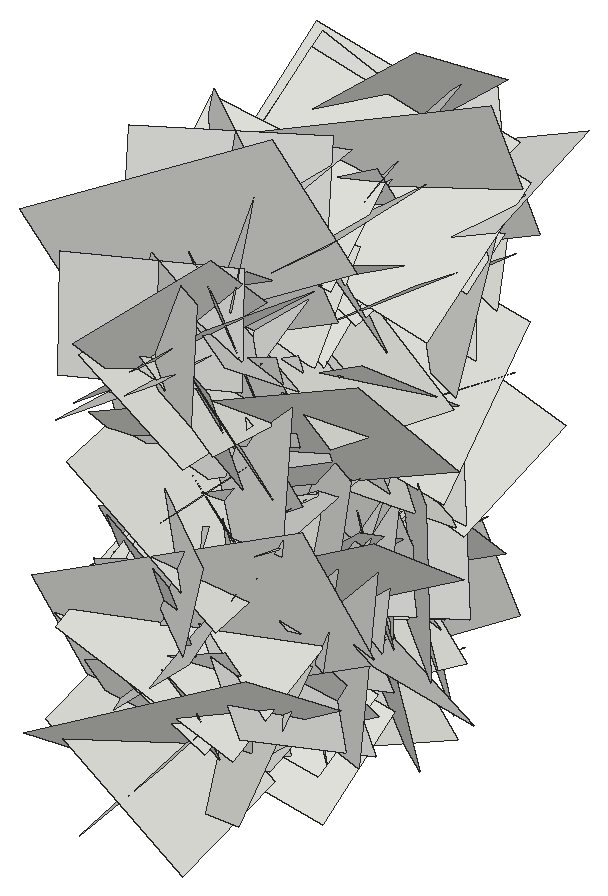
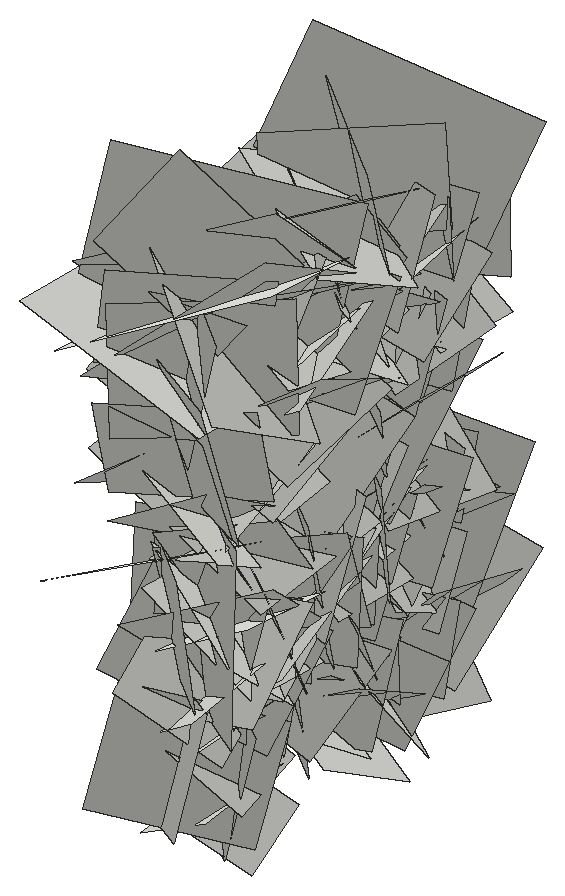
# SketchUp Ruby script. Lengths in inches.
U = 1.inch
M = Sketchup.active_model
def pt(a) = Geom::Point3d.new(a.map { |v| v * U })
def face(e, loops, mat)
  f = e.add_face(loops[0].map { |a| pt(a) })
  loops[1..].each { |l| e.add_face(l.map { |a| pt(a) }).erase! }
  f.material = f.back_material = mat if mat
  f
end
# faces: each face lists its corners as indices into pts; further lists are holes
def faces(e, pts, list, mat = nil) = list.each { |f| face(e, (f[0].is_a?(Array) ? f : [f]).map { |l| l.map { |i| pts[i] } }, mat) }
# xy, xz, yz: faces in a plane at the given z, y or x. An outline is a flat list of corners, or four numbers for a rectangle; further outlines are holes
def ring(l) = l.size == 4 ? [[l[0], l[1]], [l[2], l[1]], [l[2], l[3]], [l[0], l[3]]] : l.each_slice(2).to_a
def flat(e, list, mat, &to3) = list.each { |f| face(e, (f[0].is_a?(Array) ? f : [f]).map { |l| ring(l).map { |u, v| to3.(u, v) } }, mat) }
def xy(e, z, list, mat = nil) = flat(e, list, mat) { |x, y| [x, y, z] }
def xz(e, y, list, mat = nil) = flat(e, list, mat) { |x, z| [x, y, z] }
def yz(e, x, list, mat = nil) = flat(e, list, mat) { |y, z| [x, y, z] }
def lines(e, pts, list) = list.each { |a, b| e.add_line(pt(pts[a]), pt(pts[b])) }
# prism: a flat outline (further loops are holes) pulled along v
def prism(e, loops, v, mat = nil)
  f = face(e, loops, mat); d = Geom::Vector3d.new(v.map { |x| x * U })
  f.pushpull(f.normal.samedirection?(d) ? d.length : -d.length)
end
def box(e, o, s, mat = nil) = prism(e, [[o, [o[0] + s[0], o[1], o[2]], [o[0] + s[0], o[1] + s[1], o[2]], [o[0], o[1] + s[1], o[2]]]], [0, 0, s[2]], mat)
def at(x, y, z, deg = 0) = Geom::Transformation.translation(pt([x, y, z])) * Geom::Transformation.rotation(ORIGIN, Z_AXIS, deg.degrees)
def axes(o, x, y, z) = Geom::Transformation.new([*x, 0, *y, 0, *z, 0, *pt(o).to_a, 1])
def part(name) = M.definitions.add(name)
# library, detail: a bought-in or finely detailed component or shape, given as its bounding box
def library(name, o, s) = part(name).tap { |d| box(d.entities, o, s) }
def detail(e, o, s) = box(e.add_group.entities, o, s)
def put(e, d, t, mat = nil) = e.add_instance(d, t).tap { |i| i.material = mat if mat }
def group(e, t, mat = nil) = e.add_group.tap { |g| g.transformation = t; g.material = mat if mat }.entities
root = M.entities
c1 = part("Component\#6")
p = [[0.01,0,0],[0,3.24,4.54],[4.32,3.24,4.54],[4.33,0,0]]
faces(c1.entities,p,[[0,1,2,3]])
put(root,c1,axes([34.14,153.52,29.46],[-0.08102,0.00764,-0.81457],[-0.10707,-0.81193,0.00187],[0.85682,-0.10074,-0.07679]))
put(root,c1,axes([34.14,158.01,30.39],[0.08038,-0.60995,0.00551],[-0.02253,0.00291,0.6143],[0.64618,0.07598,0.02073]))
put(root,c1,axes([34.14,151.89,27.92],[0.07457,-0.37507,-0.49968],[-0.035,-0.50437,0.37394],[0.66135,0.0156,0.07613]))
put(root,c1,axes([38.11,158.65,23.12],[0.03,-0.65446,0.65644],[-0.11713,0.64968,0.65248],[-0.97555,-0.09812,-0.05816]))
put(root,c1,axes([34.14,150.81,32.67],[-0.03105,-0.70657,0.01303],[0.00041,0.01303,0.70717],[0.74909,-0.02929,0.00015]))
put(root,c1,axes([38.11,155.99,38.05],[-0.0315,0.52335,-0.79271],[0.01447,-0.79278,-0.52391],[-1.00678,-0.02777,0.01727]))
put(root,c1,axes([34.14,155.3,36.05],[-0.02231,-0.46484,-0.62566],[-0.10069,-0.6197,0.4636],[0.82005,-0.08874,0.0399]))
put(root,c1,axes([38.11,160.9375,37.33],[-0.13153,0.12633,-0.90974],[0.10231,-0.91113,-0.13969],[-0.96819,-0.11344,0.10882]))
put(root,c1,axes([38.11,153.79,24.7],[0.00565,-0.43188,0.90191],[0.04751,0.90112,0.43124],[-1.05892,0.03812,0.02416]))
put(root,c1,axes([38.11,152.27,30.34],[-0.04267,0.47891,-0.74389],[-0.05776,-0.74459,-0.47642],[-0.93603,0.02411,0.06331]))
put(root,c1,axes([38.11,150.92,33.45],[0.01124,-0.40239,0.85237],[-0.02564,0.85203,0.40253],[-0.99881,-0.0264,-0.00074]))
put(root,c1,axes([34.14,153.82,25.23],[0.04726,-0.11023,0.59197],[0.093,0.58845,0.10297],[0.63147,-0.07841,-0.05947]))
put(root,c1,axes([34.14,149.71,29.1],[0.04042,0.22115,-0.567],[0.10046,-0.56334,-0.21335],[0.63725,0.07479,0.0696]))
put(root,c1,axes([38.11,154.45,36.57],[-0.07713,0.81709,0.22722],[-0.03645,0.22503,-0.82021],[-0.89825,-0.07929,0.01378]))
put(root,c1,axes([34.14,158.75,26.14],[0.12859,0.59437,-0.23179],[-0.06253,-0.22448,-0.60651],[0.67335,-0.13435,-0.01206]))
put(root,c1,axes([38.11,156.72,22.08],[0.00521,-0.94479,0.50901],[0.17637,0.50353,0.93301],[-1.12382,0.07464,0.14878]))
put(root,c1,axes([34.14,156.34,37.48],[-0.20366,-0.78098,-0.33642],[0.07649,-0.35863,0.79133],[0.89812,-0.14656,-0.14368]))
put(root,c1,axes([38.11,150.56,37.37],[-0.01495,0.72639,-0.4873],[-0.06872,-0.48689,-0.7239],[-0.92463,0.02444,0.06168]))
put(root,c1,axes([34.14,156.49,28.09],[0.01227,0.36562,0.53928],[0.0952,0.53332,-0.36351],[0.68404,-0.08079,0.04092]))
put(root,c1,axes([38.11,150.4,30.92],[-0.04252,-0.27759,0.76161],[-0.13298,0.75548,0.26875],[-0.84891,-0.10444,-0.08025]))
put(root,c1,axes([38.11,152.31,24.83],[-0.14132,0.38772,0.61473],[-0.11706,0.60692,-0.40674],[-0.76145,-0.16526,-0.05156]))
put(root,c1,axes([34.14,150.69,21.46],[-0.08617,-0.06424,0.73191],[0.1147,0.7273,0.07585],[0.77031,-0.11548,0.07058]))
put(root,c1,axes([34.14,149.63,26.39],[-0.05575,0.3601,-0.58557],[0.15834,-0.56726,-0.36226],[0.71127,0.15451,0.03475]))
put(root,c1,axes([34.14,153.92,21.15],[-0.0271,-0.2919,0.8704],[-0.20523,0.85287,0.28034],[0.95124,0.17569,0.08528]))
put(root,c1,axes([34.14,159.1875,20.3125],[-0.01409,-0.35632,0.80543],[-0.16766,0.79339,0.34838],[0.91839,0.13938,0.07596]))
put(root,c1,axes([38.11,157.73,31.39],[0.13129,-0.92283,0.37392],[-0.04334,0.37177,0.93107],[-1.05456,-0.13017,0.00829]))
put(root,c1,axes([34.14,147.16,24.1],[-0.03025,0.92414,0.23442],[-0.23339,0.2218,-0.90118],[0.98329,0.08108,-0.20669]))
put(root,c1,axes([34.14,159.76,21.63],[0.09665,-0.666,0.12875],[-0.03078,0.12595,0.67212],[0.71837,0.095,0.01147]))
put(root,c1,axes([38.11,154.61,36.92],[0.07328,1.03426,0.55463],[0.26621,0.52968,-1.01904],[-1.21518,0.17841,-0.1898]))
put(root,c1,axes([34.14,160.84,30.26],[0.09118,-0.56201,-0.30691],[0.0596,-0.30185,0.56849],[0.67615,0.1024,-0.00872]))
put(root,c1,axes([34.14,156.05,22.34],[0.04217,-0.56806,-0.37659],[0.07293,-0.37196,0.56834],[0.71876,0.07107,-0.03557]))
put(root,c1,axes([38.11,158.82,28.52],[0.0834,-0.34729,-0.88838],[-0.00654,-0.89156,0.34799],[-1.01106,-0.02288,-0.07553]))
put(root,c1,axes([38.11,151.53,22],[0.08087,0.78957,0.40941],[-0.10212,0.41583,-0.78401],[-0.93722,0.02282,0.12075]))
put(root,c1,axes([38.11,152.86,25.21],[-0.07237,-0.84668,-0.40971],[0.16913,-0.41526,0.83156],[-0.98259,-0.00911,0.17331]))
put(root,c1,axes([38.11,150.44,37.52],[0.01758,-0.03984,-0.83316],[-0.08726,-0.82933,0.03802],[-0.87984,0.08145,-0.02042]))
put(root,c1,axes([38.11,161.57,34.4],[0.05292,-0.24359,-0.78611],[-0.1523,-0.77804,0.23197],[-0.85897,0.12294,-0.08956]))
put(root,c1,axes([34.14,154.14,39.875],[-0.07687,-0.17009,-0.90128],[-0.07958,-0.89996,0.17589],[0.96896,-0.0874,-0.05706]))
put(root,c1,axes([34.14,159.35,19.53],[0.12506,-0.65018,0.20227],[-0.00025,0.20525,0.65988],[0.72178,0.11273,-0.03482]))
put(root,c1,axes([38.11,155.63,34.51],[0.04715,-0.7148,-0.47013],[-0.06325,-0.47221,0.71232],[-0.90467,-0.00424,-0.0743]))
put(root,c1,axes([38.11,151.43,29.49],[0.01376,0.93036,0.01045],[0.09599,0.00914,-0.92605],[-0.98156,0.01394,-0.09041]))
put(root,c1,axes([38.11,156.02,27.27],[-0.01737,0.78195,0.05447],[-0.0729,0.05284,-0.77921],[-0.82768,-0.02106,0.06749]))
put(root,c1,axes([34.14,152.23,36.27],[0.17612,0.33723,0.58016],[-0.03508,0.60107,-0.33991],[0.71045,-0.05392,-0.16061]))
put(root,c1,axes([34.14,152.86,32.22],[-0.07765,-0.95123,0.12327],[-0.10469,0.13045,0.94796],[1.01133,-0.05954,0.1076]))
put(root,c1,axes([38.11,160.42,26.72],[0.04031,-0.6417,-0.5437],[-0.04231,-0.54502,0.64047],[-0.89052,-0.00315,-0.05504]))
put(root,c1,axes([34.14,153.18,27.99],[-0.08911,-1.01671,-0.11332],[-0.1646,-0.0997,1.00972],[1.07181,-0.09984,0.14565]))
put(root,c1,axes([38.11,153.18,27.99],[0.08911,-1.01671,-0.11332],[0.1646,-0.0997,1.00972],[-1.07181,-0.09984,0.14565]))
put(root,c1,axes([34.14,160.42,26.72],[-0.04031,-0.6417,-0.5437],[0.04231,-0.54502,0.64047],[0.89052,-0.00315,-0.05504]))
put(root,c1,axes([38.11,152.86,32.22],[0.07765,-0.95123,0.12327],[0.10469,0.13045,0.94796],[-1.01133,-0.05954,0.1076]))
put(root,c1,axes([38.11,152.23,36.27],[-0.17612,0.33723,0.58016],[0.03508,0.60107,-0.33991],[-0.71045,-0.05392,-0.16061]))
put(root,c1,axes([34.14,156.02,27.27],[0.01737,0.78195,0.05447],[0.0729,0.05284,-0.77921],[0.82768,-0.02106,0.06749]))
put(root,c1,axes([34.14,151.43,29.49],[-0.01376,0.93036,0.01045],[-0.09599,0.00914,-0.92605],[0.98156,0.01394,-0.09041]))
put(root,c1,axes([34.14,155.63,34.51],[-0.04715,-0.7148,-0.47013],[0.06325,-0.47221,0.71232],[0.90467,-0.00424,-0.0743]))
put(root,c1,axes([38.11,159.35,19.53],[-0.12506,-0.65018,0.20227],[0.00025,0.20525,0.65988],[-0.72178,0.11273,-0.03482]))
put(root,c1,axes([38.11,154.14,39.875],[0.07687,-0.17009,-0.90128],[0.07958,-0.89996,0.17589],[-0.96896,-0.0874,-0.05706]))
put(root,c1,axes([34.14,161.57,34.4],[-0.05292,-0.24359,-0.78611],[0.1523,-0.77804,0.23197],[0.85897,0.12294,-0.08956]))
put(root,c1,axes([34.14,150.44,37.52],[-0.01758,-0.03984,-0.83316],[0.08726,-0.82933,0.03802],[0.87984,0.08145,-0.02042]))
put(root,c1,axes([34.14,152.86,25.21],[0.07237,-0.84668,-0.40971],[-0.16913,-0.41526,0.83156],[0.98259,-0.00911,0.17331]))
put(root,c1,axes([34.14,151.53,22],[-0.08087,0.78957,0.40941],[0.10212,0.41583,-0.78401],[0.93722,0.02282,0.12075]))
put(root,c1,axes([34.14,158.82,28.52],[-0.0834,-0.34729,-0.88838],[0.00654,-0.89156,0.34799],[1.01106,-0.02288,-0.07553]))
put(root,c1,axes([38.11,156.05,22.34],[-0.04217,-0.56806,-0.37659],[-0.07293,-0.37196,0.56834],[-0.71876,0.07107,-0.03557]))
put(root,c1,axes([38.11,160.84,30.26],[-0.09118,-0.56201,-0.30691],[-0.0596,-0.30185,0.56849],[-0.67615,0.1024,-0.00872]))
put(root,c1,axes([34.14,154.61,36.92],[-0.07328,1.03426,0.55463],[-0.26621,0.52968,-1.01904],[1.21518,0.17841,-0.1898]))
put(root,c1,axes([38.11,159.76,21.63],[-0.09665,-0.666,0.12875],[0.03078,0.12595,0.67212],[-0.71837,0.095,0.01147]))
put(root,c1,axes([38.11,147.16,24.1],[0.03025,0.92414,0.23442],[0.23339,0.2218,-0.90118],[-0.98329,0.08108,-0.20669]))
put(root,c1,axes([34.14,157.73,31.39],[-0.13129,-0.92283,0.37392],[0.04334,0.37177,0.93107],[1.05456,-0.13017,0.00829]))
put(root,c1,axes([38.11,159.1875,20.3125],[0.01409,-0.35632,0.80543],[0.16766,0.79339,0.34838],[-0.91839,0.13938,0.07596]))
put(root,c1,axes([38.11,153.92,21.15],[0.0271,-0.2919,0.8704],[0.20523,0.85287,0.28034],[-0.95124,0.17569,0.08528]))
put(root,c1,axes([38.11,149.63,26.39],[0.05575,0.3601,-0.58557],[-0.15834,-0.56726,-0.36226],[-0.71127,0.15451,0.03475]))
put(root,c1,axes([38.11,150.69,21.46],[0.08617,-0.06424,0.73191],[-0.1147,0.7273,0.07585],[-0.77031,-0.11548,0.07058]))
put(root,c1,axes([34.14,152.31,24.83],[0.14132,0.38772,0.61473],[0.11706,0.60692,-0.40674],[0.76145,-0.16526,-0.05156]))
put(root,c1,axes([34.14,150.4,30.92],[0.04252,-0.27759,0.76161],[0.13298,0.75548,0.26875],[0.84891,-0.10444,-0.08025]))
put(root,c1,axes([38.11,156.49,28.09],[-0.01227,0.36562,0.53928],[-0.0952,0.53332,-0.36351],[-0.68404,-0.08079,0.04092]))
put(root,c1,axes([34.14,150.56,37.37],[0.01495,0.72639,-0.4873],[0.06872,-0.48689,-0.7239],[0.92463,0.02444,0.06168]))
put(root,c1,axes([38.11,156.34,37.48],[0.20366,-0.78098,-0.33642],[-0.07649,-0.35863,0.79133],[-0.89812,-0.14656,-0.14368]))
put(root,c1,axes([34.14,156.72,22.08],[-0.00521,-0.94479,0.50901],[-0.17637,0.50353,0.93301],[1.12382,0.07464,0.14878]))
put(root,c1,axes([38.11,158.75,26.14],[-0.12859,0.59437,-0.23179],[0.06253,-0.22448,-0.60651],[-0.67335,-0.13435,-0.01206]))
put(root,c1,axes([34.14,154.45,36.57],[0.07713,0.81709,0.22722],[0.03645,0.22503,-0.82021],[0.89825,-0.07929,0.01378]))
put(root,c1,axes([38.11,149.71,29.1],[-0.04042,0.22115,-0.567],[-0.10046,-0.56334,-0.21335],[-0.63725,0.07479,0.0696]))
put(root,c1,axes([38.11,153.82,25.23],[-0.04726,-0.11023,0.59197],[-0.093,0.58845,0.10297],[-0.63147,-0.07841,-0.05947]))
put(root,c1,axes([34.14,150.92,33.45],[-0.01124,-0.40239,0.85237],[0.02564,0.85203,0.40253],[0.99881,-0.0264,-0.00074]))
put(root,c1,axes([34.14,152.27,30.34],[0.04267,0.47891,-0.74389],[0.05776,-0.74459,-0.47642],[0.93603,0.02411,0.06331]))
put(root,c1,axes([34.14,153.79,24.7],[-0.00565,-0.43188,0.90191],[-0.04751,0.90112,0.43124],[1.05892,0.03812,0.02416]))
put(root,c1,axes([34.14,160.9375,37.33],[0.13153,0.12633,-0.90974],[-0.10231,-0.91113,-0.13969],[0.96819,-0.11344,0.10882]))
put(root,c1,axes([38.11,155.3,36.05],[0.02231,-0.46484,-0.62566],[0.10069,-0.6197,0.4636],[-0.82005,-0.08874,0.0399]))
put(root,c1,axes([34.14,155.99,38.05],[0.0315,0.52335,-0.79271],[-0.01447,-0.79278,-0.52391],[1.00678,-0.02777,0.01727]))
put(root,c1,axes([38.11,150.81,32.67],[0.03105,-0.70657,0.01303],[-0.00041,0.01303,0.70717],[-0.74909,-0.02929,0.00015]))
put(root,c1,axes([34.14,158.65,23.12],[-0.03,-0.65446,0.65644],[0.11713,0.64968,0.65248],[0.97555,-0.09812,-0.05816]))
put(root,c1,axes([38.11,151.89,27.92],[-0.07457,-0.37507,-0.49968],[0.035,-0.50437,0.37394],[-0.66135,0.0156,0.07613]))
put(root,c1,axes([38.11,158.01,30.39],[-0.08038,-0.60995,0.00551],[0.02253,0.00291,0.6143],[-0.64618,0.07598,0.02073]))
put(root,c1,axes([38.11,153.52,29.46],[0.08102,0.00764,-0.81457],[0.10707,-0.81193,0.00187],[-0.85682,-0.10074,-0.07679]))
put(root,c1,axes([34.14,152.65,32.7],[-0.31384,1.21799,0.62272],[-0.13011,0.61092,-1.25326],[1.44417,0.31973,0.02242]))
put(root,c1,axes([34.14,149.65,34.23],[-0.2234,-0.54463,1.08834],[-0.02633,1.10624,0.54877],[1.28976,-0.07175,0.19972]))
put(root,c1,axes([38.11,152.7,33.94],[0.15183,0.13661,-0.74127],[-0.04087,-0.75222,-0.14607],[-0.79793,0.06452,-0.13357]))
put(root,c1,axes([38.11,158.73,27.09],[0.13155,-0.14233,-0.74779],[0.00006,-0.75766,0.14422],[-0.80689,-0.02326,-0.12191]))
put(root,c1,axes([34.14,158.66,27.8],[0.19419,0.10037,-0.91545],[-0.10975,-0.92523,-0.12216],[0.97001,-0.12478,0.16945]))
put(root,c1,axes([38.11,156.65,23.33],[-0.01341,0.01203,0.69899],[0.10657,0.69187,-0.01009],[-0.73333,0.10033,-0.01425]))
put(root,c1,axes([34.14,154.96,37.56],[-0.27688,1.1515,0.31839],[0.11464,0.34737,-1.16756],[1.26119,0.22122,0.17603]))
put(root,c1,axes([34.14,152.42,20.54],[-0.05004,-0.6691,0.77955],[0.05919,0.77755,0.67076],[1.08735,-0.07312,-0.00064]))
put(root,c1,axes([38.11,161,38.46],[0.19651,-0.13504,-0.81499],[0.03185,-0.8336,0.14496],[-0.87508,-0.06067,-0.17773]))
put(root,c1,axes([34.14,159.15,23.91],[0.14407,0.13595,-0.90237],[-0.02833,-0.91134,-0.14133],[0.9669,-0.04696,0.13032]))
put(root,c1,axes([34.14,151.25,34.8],[0.16779,0.3958,-0.75565],[0.05631,-0.77163,-0.39305],[0.90246,-0.02545,0.16502]))
put(root,c1,axes([38.11,158.03,24.73],[0.19324,-0.05037,0.89121],[0.15909,0.89838,0.02008],[-0.93272,0.1428,0.18806]))
put(root,c1,axes([34.14,154.4,23.625],[-0.0407,-0.65785,-0.83395],[0.03781,-0.83482,0.65689],[1.12528,0.00426,-0.05223]))
put(root,c1,axes([38.11,157.59,40.82],[0.16311,0.68993,-0.43022],[0.09586,-0.44966,-0.68876],[-0.85651,0.08106,-0.15901]))
put(root,c1,axes([34.14,154.59,24.16],[-0.1724,0.15274,1.09758],[0.17194,1.10067,-0.12914],[1.16199,-0.14021,0.18195]))
put(root,c1,axes([34.14,152.14,28.92],[0.00837,0.82237,-0.50147],[0.16225,-0.49618,-0.8113],[1.00803,0.07304,0.13474]))
put(root,c1,axes([38.11,149.08,38.35],[-0.0057,0.54335,-0.52891],[0.23788,-0.50408,-0.52014],[-0.76776,-0.16022,-0.15723]))
put(root,c1,axes([38.11,157.4,31.875],[0.05779,-0.51798,-0.36432],[0.0587,-0.36037,0.52065],[-0.6687,-0.0764,0.01422]))
put(root,c1,axes([34.14,156.45,32.24],[0.14884,0.843,-0.57449],[-0.06248,-0.57223,-0.85409],[1.07954,-0.14935,0.02978]))
put(root,c1,axes([38.11,160.09,33.87],[0.13785,-0.16653,-0.67513],[0.04892,-0.68326,0.17743],[-0.73546,-0.07666,-0.11474]))
put(root,c1,axes([34.14,156.02,28.65],[-0.0619,-0.85924,0.62732],[0.17366,0.61351,0.85557],[1.11425,-0.14335,-0.09849]))
put(root,c1,axes([38.11,147.9,27.03],[0.12769,0.03013,0.63893],[0.01482,0.64988,-0.03329],[-0.67785,0.01989,0.11963]))
put(root,c1,axes([34.14,156.69,29.48],[-0.02364,1.01192,0.31394],[0.16386,0.31376,-1.00035],[1.11105,-0.02474,0.15421]))
put(root,c1,axes([34.14,161.68,35.57],[-0.09547,-0.29138,-1.10436],[0.14499,-1.10257,0.27976],[1.20197,0.10985,-0.12146]))
put(root,c1,axes([34.14,147.58,26.68],[0.22766,0.71104,0.67114],[-0.02672,0.69094,-0.72395],[1.03608,-0.13842,-0.16614]))
put(root,c1,axes([34.14,153.43,27.14],[0.15407,-0.97446,-0.01303],[0.08051,-0.00181,0.98239],[1.02988,0.14592,-0.07485]))
put(root,c1,axes([34.14,158.93,27.77],[-0.0679,-1.16178,0.21088],[0.08573,0.20637,1.16154],[1.24867,-0.07734,-0.06828]))
put(root,c1,axes([34.14,160.05,30.35],[-0.12426,0.20575,-1.35522],[-0.11745,-1.35714,-0.19646],[1.44825,-0.0924,-0.13221]))
put(root,c1,axes([34.14,157.84,26.69],[0.16666,-0.37984,-0.88441],[0.10341,-0.88523,0.39754],[1.01503,0.15255,0.10471]))
put(root,c1,axes([34.14,153.58,31.99],[0.17505,-0.32324,-0.90395],[0.10086,-0.9072,0.34179],[1.0126,0.14624,0.12223]))
put(root,c1,axes([34.14,151.45,29.33],[0.11063,1.17252,-0.59491],[-0.28501,-0.56514,-1.16101],[1.36425,-0.21315,-0.19431]))
put(root,c1,axes([34.14,155.57,33.875],[0.13701,-1.11756,0.11199],[-0.07264,0.10468,1.12363],[1.18833,0.13525,0.05577]))
put(root,c1,axes([34.14,156.79,29.67],[0.01777,-0.29003,-1.18393],[-0.05362,-1.18318,0.28913],[1.29096,-0.04516,0.0283]))
put(root,c1,axes([34.14,158.37,30.5],[0.12568,-1.12455,0.31778],[-0.06348,0.31314,1.13049],[1.23707,0.13032,0.02572]))
put(root,c1,axes([34.14,152.25,36.24],[-0.0137,1.21221,-0.26433],[0.01965,-0.26413,-1.21218],[1.31499,0.01657,0.01536]))
put(root,c1,axes([34.14,150.2,21.48],[0.03659,-0.96074,0.6365],[0.08804,0.6372,0.9573],[1.21843,-0.01719,-0.08829]))
put(root,c1,axes([34.14,149.67,23.37],[-0.09539,-0.59855,1.14231],[0.08783,1.14003,0.60389],[1.36418,-0.11525,0.041]))
put(root,c1,axes([34.14,153.92,36.42],[0.14295,0.82362,0.79821],[0.11339,0.79118,-0.83443],[1.21047,-0.17138,-0.0161]))
put(root,c1,axes([34.14,156.14,33.68],[0.06217,-0.55405,1.15944],[0.03014,1.16092,0.55332],[1.36179,-0.0004,-0.06518]))
put(root,c1,axes([34.14,157.5625,26.25],[0.15158,-0.38022,-1.22414],[-0.0526,-1.23246,0.37701],[1.35773,-0.0053,0.15127]))
put(root,c1,axes([34.14,161.74,34.71],[0.1652,-1.10091,-0.16395],[0.26327,-0.12698,1.08875],[1.15009,0.1872,-0.22568]))
put(root,c1,axes([34.14,153.73,28.3],[-0.01858,0.99462,-0.84655],[0.29457,-0.8244,-0.97435],[1.35277,0.19318,0.20054]))
put(root,c1,axes([34.14,153.125,28.17],[-0.03085,-0.9293,0.97672],[0.26234,0.95667,0.91759],[1.40479,-0.19906,-0.14991]))
put(root,c1,axes([34.14,153.14,23.91],[0.18,-1.08552,0.79109],[0.08355,0.80406,1.08641],[1.42134,0.0902,-0.16405]))
